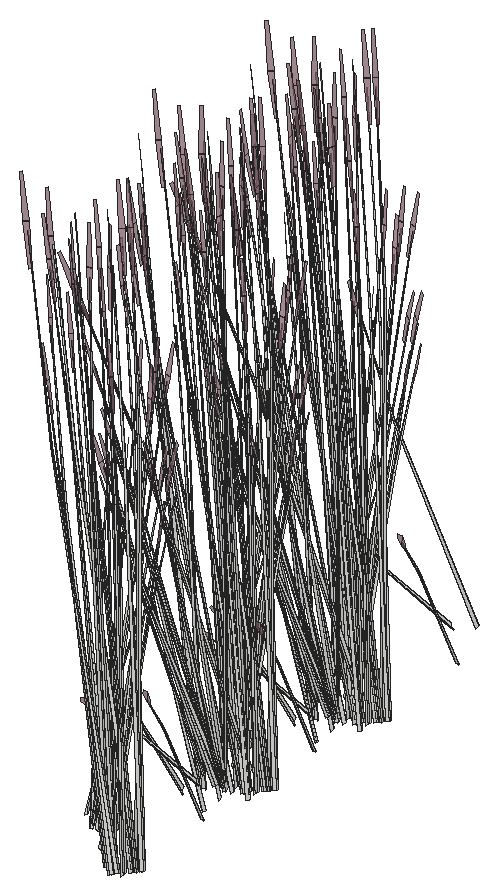
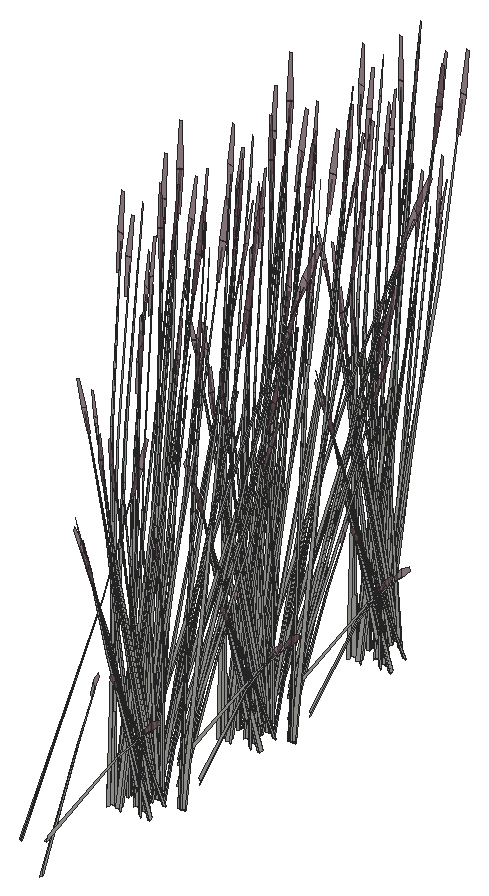
# SketchUp Ruby script. Lengths in inches.
U = 1.inch
M = Sketchup.active_model
def pt(a) = Geom::Point3d.new(a.map { |v| v * U })
def face(e, loops, mat)
  f = e.add_face(loops[0].map { |a| pt(a) })
  loops[1..].each { |l| e.add_face(l.map { |a| pt(a) }).erase! }
  f.material = f.back_material = mat if mat
  f
end
# faces: each face lists its corners as indices into pts; further lists are holes
def faces(e, pts, list, mat = nil) = list.each { |f| face(e, (f[0].is_a?(Array) ? f : [f]).map { |l| l.map { |i| pts[i] } }, mat) }
# xy, xz, yz: faces in a plane at the given z, y or x. An outline is a flat list of corners, or four numbers for a rectangle; further outlines are holes
def ring(l) = l.size == 4 ? [[l[0], l[1]], [l[2], l[1]], [l[2], l[3]], [l[0], l[3]]] : l.each_slice(2).to_a
def flat(e, list, mat, &to3) = list.each { |f| face(e, (f[0].is_a?(Array) ? f : [f]).map { |l| ring(l).map { |u, v| to3.(u, v) } }, mat) }
def xy(e, z, list, mat = nil) = flat(e, list, mat) { |x, y| [x, y, z] }
def xz(e, y, list, mat = nil) = flat(e, list, mat) { |x, z| [x, y, z] }
def yz(e, x, list, mat = nil) = flat(e, list, mat) { |y, z| [x, y, z] }
def lines(e, pts, list) = list.each { |a, b| e.add_line(pt(pts[a]), pt(pts[b])) }
# prism: a flat outline (further loops are holes) pulled along v
def prism(e, loops, v, mat = nil)
  f = face(e, loops, mat); d = Geom::Vector3d.new(v.map { |x| x * U })
  f.pushpull(f.normal.samedirection?(d) ? d.length : -d.length)
end
def box(e, o, s, mat = nil) = prism(e, [[o, [o[0] + s[0], o[1], o[2]], [o[0] + s[0], o[1] + s[1], o[2]], [o[0], o[1] + s[1], o[2]]]], [0, 0, s[2]], mat)
def at(x, y, z, deg = 0) = Geom::Transformation.translation(pt([x, y, z])) * Geom::Transformation.rotation(ORIGIN, Z_AXIS, deg.degrees)
def axes(o, x, y, z) = Geom::Transformation.new([*x, 0, *y, 0, *z, 0, *pt(o).to_a, 1])
def part(name) = M.definitions.add(name)
# library, detail: a bought-in or finely detailed component or shape, given as its bounding box
def library(name, o, s) = part(name).tap { |d| box(d.entities, o, s) }
def detail(e, o, s) = box(e.add_group.entities, o, s)
def put(e, d, t, mat = nil) = e.add_instance(d, t).tap { |i| i.material = mat if mat }
def group(e, t, mat = nil) = e.add_group.tap { |g| g.transformation = t; g.material = mat if mat }.entities
root = M.entities
M.materials.add("LightPink_Translucent").color = [144, 107, 117]
M.materials["LightPink_Translucent"].alpha = 0.75
c1 = part("blade")
p = [[2.15,0.21,22],[0,0.17,0],[0.09,0.45,0],[2.18,0.31,22],[2.29,0.31,22],[0.38,0.45,0],
  [2.48,0.24,33],[2.49,0.24,33],[2.48,0.22,33]]
faces(c1.entities,p,[[0,1,2,3],[4,5,2,3],[6,3,4,7],[8,0,3,6]])
c2 = part("seeds")
p = [[0.3,-0.1,1.38],[-0.01,-0.03,1.59],[-0.01,-0.03,0.03],[0.14,-0.07,-0.07],[0.29,-0.03,3],[0.15,0.01,3.11]]
faces(c2.entities,p,[[0,1,2,3],[1,0,4,5]],"LightPink_Translucent")
c3 = part("blade with seeds")
put(c3.entities,c1,at(0,0,0))
put(c3.entities,c2,axes([2.4,0.25,30.99],[1.5799,-0.05474,1.17369],[-0.12525,1.92788,0.29478],[-0.07173,-0.02425,1.56792]))
put(root,c3,axes([343.19,119.87,4.77],[0.96132,-0.17317,0.17642],[0.23737,0.64447,0.35086],[-0.08574,-0.0939,1.60407]))
put(root,c3,axes([344.08,119.18,4.91],[-0.17258,0.58229,0.1448],[-0.84319,-0.10108,-0.41347],[-0.15345,-0.05979,1.26744]))
put(root,c3,axes([346.05,119.9,4.77],[0.25843,-0.64844,0.17642],[0.9457,0.1835,0.35086],[-0.16336,0.00316,1.60407]))
put(root,c3,axes([344.43,119.97,4.49],[-0.90188,-0.29293,0],[0.43405,-0.60866,0],[0,0,1.62707]))
put(root,c3,axes([345.18,119.19,4.76],[-0.87356,-0.52515,-0.25192],[0.73507,-0.5897,0.5513],[-0.23523,0.06143,1.68216]))
put(root,c3,axes([342.88,120.2,4.77],[0.83726,0.32623,0.49651],[-0.50045,0.58498,0],[-0.19069,-0.0743,1.57504]))
put(root,c3,axes([345.6,118.76,5.01],[0.97146,-0.04028,0.44739],[0.08785,0.66859,-0.21531],[-0.17391,0.06776,1.43643]))
put(root,c3,axes([344.74,119.08,4.5],[-0.97146,0.04028,-0.44739],[-0.08785,-0.66859,0.21531],[-0.17391,0.06776,1.43643]))
put(root,c3,axes([345.8125,120.63,4.49],[-0.55235,-0.65609,-0.05142],[0.93577,-0.36461,0.51607],[-0.23059,0.06247,1.6363]))
put(root,c3,axes([345.62,119.04,4.91],[0.66093,0.39201,0.1448],[-0.5513,0.44227,-0.41347],[-0.15345,0.05979,1.26744]))
put(root,c3,axes([346.32,120.25,4.77],[0.83726,-0.32623,0.49651],[0.50045,0.58498,0],[-0.19069,0.0743,1.57504]))
put(root,c3,axes([345.5625,120.55,4.32],[-0.83462,-0.16144,-0.30978],[0.21015,-0.56852,0.30978],[-0.16826,0.06556,1.38974]))
put(root,c3,axes([345.42,118.9,4.96],[0.10425,0.7445,-0.29095],[-1.08575,0.04502,-0.50002],[-0.19119,0.09917,1.59708]))
put(root,c3,axes([344.77,119.47,4.35],[-0.60257,0.49041,-0.62353],[-0.74854,-0.44469,-0.16365],[-0.24146,0.12234,1.37633]))
put(root,c3,axes([345.84,120.29,4.625],[1.11998,0.21207,0.30756],[-0.2802,0.75803,-0.36492],[-0.18537,0.09487,1.64885]))
put(root,c3,axes([345.76,120.8,4.3125],[-0.83726,0.32623,-0.49651],[-0.50045,-0.58498,0],[-0.19069,0.0743,1.57504]))
put(root,c3,axes([341.98,120.01,7.34],[0.60531,-0.34352,0.35414],[0.573,0.39225,-0.4572],[-0.08718,0.19929,0.87481]))
put(root,c3,axes([346.52,120.7,4.67],[0.55932,0.6538,0],[-0.93577,0.36461,-0.51607],[-0.21313,0.08304,1.63711]))
put(root,c3,axes([346.04,118.12,5.13],[-0.02444,-0.61432,1.41272],[1.10603,0.15924,0.59816],[-0.26159,0.33615,1.3335]))
put(root,c3,axes([343.4375,121.03,7.02],[-0.6592,0.22175,0.0643],[-0.32265,-0.40436,0.50621],[0.06366,0.17825,0.77189]))
put(root,c3,axes([341.67,120.49,6.82],[-0.60531,0.34352,-0.35414],[-0.573,-0.39225,0.4572],[-0.08718,0.19929,0.87481]))
put(root,c3,axes([341.6,120.1,7.69],[0.98321,0.03233,-0.13498],[-0.02687,0.61208,-0.74919],[-0.0683,0.23574,1.13838]))
put(root,c3,axes([343.67,120.98,7.36],[-0.88151,-0.17057,0.53283],[0.30143,-0.56078,0.43934],[0.05297,0.22053,1.10256]))
put(root,c3,axes([342.05,121.83,5.06],[-0.02315,-0.38796,1.1486],[0.57853,0.27671,0.84392],[-0.11378,0.18492,0.25299]))
put(root,c3,axes([342.27,120.33,7.3],[0.64041,0.4384,-0.5672],[-0.67652,0.38394,-0.43934],[-0.09744,0.22274,1.08528]))
put(root,c3,axes([341.57,120.99,5.12],[0.8127,-0.11554,0.06507],[0.18684,0.46549,-0.86304],[-0.05152,0.23564,0.7736]))
put(root,c3,axes([342.07,120.13,7.63],[-0.02328,0.60353,-0.7886],[-0.98022,-0.04053,0.09517],[-0.10344,0.25568,1.11556]))
put(root,c3,axes([339.51,121.72,7],[0.10149,-0.03939,1.77383],[0.83886,0.26202,-0.16761],[-0.01971,0.21816,0.31391]))
put(root,c3,axes([343,119.7,6.17],[-0.0219,-0.25042,1.71376],[0.94901,0.16613,0.13857],[-0.0587,0.35688,0.73262]))
put(root,c3,axes([343.98,131.05,7.01],[-0.13683,-0.09148,1.74944],[-0.91315,0.058,-0.27667],[-0.14574,-0.2188,0.14031]))
put(root,c3,axes([341.74,120.98,5.66],[0.01966,-0.33682,1.54345],[0.88405,0.17791,0.21329],[-0.0766,0.35897,0.72882]))
put(root,c3,axes([344.94,132.59,7.27],[-0.42698,-0.53052,-0.71045],[0.87893,-0.29566,0.08574],[-0.09984,-0.25633,1.00501]))
put(root,c3,axes([344.2,131.42,3.79],[-0.15005,0.02351,1.76342],[-0.82981,-0.26461,-0.26939],[0.01392,-0.22072,0.30037]))
put(root,c3,axes([345.02,132.14,6.82],[0.2697,-0.50175,-0.35414],[0.78684,0.14635,0.4572],[-0.07215,-0.20201,0.87481]))
put(root,c3,axes([344.62,132.49,6.97],[-0.87941,-0.16356,-0.51099],[0.30143,-0.56078,-0.3958],[-0.08064,-0.22578,0.97773]))
put(root,c3,axes([342.87,132.14,7.39],[0.99656,-0.1677,0.53763],[0.17295,0.65785,0.4433],[-0.23438,-0.19388,1.11249]))
put(root,c3,axes([345.37,132.46,7.33],[-0.87543,0.30377,-0.1216],[-0.4302,-0.53915,-0.67495],[-0.1155,-0.2272,1.02557]))
put(root,c3,axes([341.89,131.54,5.06],[0.46666,0.22709,1.1486],[-0.67962,0.13651,0.84392],[-0.14541,-0.17452,0.25299]))
put(root,c3,axes([343.09,132.28,7.02],[0.4066,-0.41448,0.0643],[0.57901,0.24131,0.50621],[-0.18719,-0.13288,0.77189]))
put(root,c3,axes([342.97,134.59,4.39],[-0.36739,-0.66907,-0.69835],[1.05831,-0.24096,-0.18329],[-0.04061,-0.22656,1.54149]))
put(root,c3,axes([345.11,132.67,7.34],[-0.2697,0.50175,0.35414],[-0.78684,-0.14635,-0.4572],[-0.07215,-0.20201,0.87481]))
put(root,c3,axes([344.05,131.875,4.42],[-0.61821,0.37431,-0.03893],[-0.56645,-0.40995,-0.17649],[-0.03988,-0.11616,0.58215]))
put(root,c3,axes([344.84,136.3125,5.62],[0.77308,0.2631,1.51261],[-0.75736,0.56681,0.59816],[-0.33924,-0.33594,1.26806]))
put(root,c3,axes([343.22,132.76,7.34],[0.13817,0.52554,0.35414],[-0.78985,0.13877,-0.4572],[-0.21215,-0.1506,0.87481]))
put(root,c3,axes([340.8,134.49,4.3125],[0,-0.65246,-0.49651],[1.00089,0,0],[0,-0.1486,1.57504]))
put(root,c3,axes([341.23,134.51,4.32],[0.62448,-0.40708,-0.30978],[0.62448,0.40708,0.30978],[0,-0.13112,1.38974]))
put(root,c3,axes([343.42,135.25,4.96],[-1.00749,-0.31132,-0.29095],[0.48511,-0.65709,-0.50002],[-0.03166,-0.16133,1.59708]))
put(root,c3,axes([341.42,134.8,4.625],[-0.83213,0.54855,0.30756],[-0.83263,-0.54278,-0.36492],[-0.02906,-0.15578,1.64885]))
put(root,c3,axes([343.67,135.94,4.73],[0.23711,-0.77313,-0.23429],[1.12425,0.13477,0.51271],[-0.19645,-0.10677,1.5644]))
put(root,c3,axes([341.23,135.1,4.77],[0,0.65246,0.49651],[-1.00089,0,0],[0,-0.1486,1.57504]))
put(root,c3,axes([343.59,135.625,4.5],[-0.53742,-0.54764,-0.44739],[0.81403,-0.38564,0.21531],[-0.17391,-0.06776,1.43643]))
put(root,c3,axes([343.7,134.85,4.65],[0.38895,0.72959,0.45755],[-1.11135,0.2537,0.17955],[0.01358,-0.13406,1.58856]))
put(root,c3,axes([343.51,135.43,5.01],[-0.43405,0.58792,0.44739],[-0.90188,-0.28295,-0.21531],[0,-0.13553,1.43643]))
put(root,c3,axes([345.38,135.5,4.59],[-0.83213,-0.56158,-0.06131],[0.83263,-0.56193,0],[-0.02906,-0.01961,1.75571]))
put(root,c3,axes([343.8,135.57,4.65],[1.13071,0.13747,0.45755],[-0.23011,0.77639,0.17955],[-0.16524,-0.07497,1.58856]))
put(root,c3,axes([343.19,136.81,4.77],[0.96132,-0.17317,0.17642],[0.23737,0.64447,0.35086],[-0.08574,-0.0939,1.60407]))
put(root,c3,axes([344.08,136.12,4.91],[-0.17258,0.58229,0.1448],[-0.84319,-0.10108,-0.41347],[-0.15345,-0.05979,1.26744]))
put(root,c3,axes([346.05,136.84,4.77],[0.25843,-0.64844,0.17642],[0.9457,0.1835,0.35086],[-0.16336,0.00316,1.60407]))
put(root,c3,axes([344.43,136.91,4.49],[-0.90188,-0.29293,0],[0.43405,-0.60866,0],[0,0,1.62707]))
put(root,c3,axes([345.18,136.13,4.76],[-0.87356,-0.52515,-0.25192],[0.73507,-0.5897,0.5513],[-0.23523,0.06143,1.68216]))
put(root,c3,axes([342.88,137.14,4.77],[0.83726,0.32623,0.49651],[-0.50045,0.58498,0],[-0.19069,-0.0743,1.57504]))
put(root,c3,axes([345.6,135.7,5.01],[0.97146,-0.04028,0.44739],[0.08785,0.66859,-0.21531],[-0.17391,0.06776,1.43643]))
put(root,c3,axes([344.74,136.02,4.5],[-0.97146,0.04028,-0.44739],[-0.08785,-0.66859,0.21531],[-0.17391,0.06776,1.43643]))
put(root,c3,axes([345.8125,137.57,4.49],[-0.55235,-0.65609,-0.05142],[0.93577,-0.36461,0.51607],[-0.23059,0.06247,1.6363]))
put(root,c3,axes([345.62,135.98,4.91],[0.66093,0.39201,0.1448],[-0.5513,0.44227,-0.41347],[-0.15345,0.05979,1.26744]))
put(root,c3,axes([346.32,137.19,4.77],[0.83726,-0.32623,0.49651],[0.50045,0.58498,0],[-0.19069,0.0743,1.57504]))
put(root,c3,axes([345.5625,137.49,4.32],[-0.83462,-0.16144,-0.30978],[0.21015,-0.56852,0.30978],[-0.16826,0.06556,1.38974]))
put(root,c3,axes([345.42,135.84,4.96],[0.10425,0.7445,-0.29095],[-1.08575,0.04502,-0.50002],[-0.19119,0.09917,1.59708]))
put(root,c3,axes([344.77,136.41,4.35],[-0.60257,0.49041,-0.62353],[-0.74854,-0.44469,-0.16365],[-0.24146,0.12234,1.37633]))
put(root,c3,axes([345.84,137.23,4.625],[1.11998,0.21207,0.30756],[-0.2802,0.75803,-0.36492],[-0.18537,0.09487,1.64885]))
put(root,c3,axes([345.76,137.74,4.3125],[-0.83726,0.32623,-0.49651],[-0.50045,-0.58498,0],[-0.19069,0.0743,1.57504]))
put(root,c3,axes([341.98,136.95,7.34],[0.60531,-0.34352,0.35414],[0.573,0.39225,-0.4572],[-0.08718,0.19929,0.87481]))
put(root,c3,axes([346.52,137.64,4.67],[0.55932,0.6538,0],[-0.93577,0.36461,-0.51607],[-0.21313,0.08304,1.63711]))
put(root,c3,axes([346.04,135.06,5.13],[-0.02444,-0.61432,1.41272],[1.10603,0.15924,0.59816],[-0.26159,0.33615,1.3335]))
put(root,c3,axes([341.4375,137.26,7.02],[-0.73517,-0.0304,0.0643],[0.02016,-0.45906,0.50621],[-0.07693,0.17585,0.77189]))
put(root,c3,axes([343.98,145.4,7.01],[-0.13683,-0.09148,1.74944],[-0.91315,0.058,-0.27667],[-0.14574,-0.2188,0.14031]))
put(root,c3,axes([343.4375,137.97,7.02],[-0.6592,0.22175,0.0643],[-0.32265,-0.40436,0.50621],[0.06366,0.17825,0.77189]))
put(root,c3,axes([341.67,137.43,6.82],[-0.60531,0.34352,-0.35414],[-0.573,-0.39225,0.4572],[-0.08718,0.19929,0.87481]))
put(root,c3,axes([344.94,146.94,7.27],[-0.42698,-0.53052,-0.71045],[0.87893,-0.29566,0.08574],[-0.09984,-0.25633,1.00501]))
put(root,c3,axes([341.6,137.04,7.69],[0.98321,0.03233,-0.13498],[-0.02687,0.61208,-0.74919],[-0.0683,0.23574,1.13838]))
put(root,c3,axes([343.67,137.92,7.36],[-0.88151,-0.17057,0.53283],[0.30143,-0.56078,0.43934],[0.05297,0.22053,1.10256]))
put(root,c3,axes([342.05,138.77,5.06],[-0.02315,-0.38796,1.1486],[0.57853,0.27671,0.84392],[-0.11378,0.18492,0.25299]))
put(root,c3,axes([344.2,145.76,3.79],[-0.15005,0.02351,1.76342],[-0.82981,-0.26461,-0.26939],[0.01392,-0.22072,0.30037]))
put(root,c3,axes([342.27,137.27,7.3],[0.64041,0.4384,-0.5672],[-0.67652,0.38394,-0.43934],[-0.09744,0.22274,1.08528]))
put(root,c3,axes([341.57,137.93,5.12],[0.8127,-0.11554,0.06507],[0.18684,0.46549,-0.86304],[-0.05152,0.23564,0.7736]))
put(root,c3,axes([345.02,146.49,6.82],[0.2697,-0.50175,-0.35414],[0.78684,0.14635,0.4572],[-0.07215,-0.20201,0.87481]))
put(root,c3,axes([344.62,146.84,6.97],[-0.87941,-0.16356,-0.51099],[0.30143,-0.56078,-0.3958],[-0.08064,-0.22578,0.97773]))
put(root,c3,axes([342.07,137.07,7.63],[-0.02328,0.60353,-0.7886],[-0.98022,-0.04053,0.09517],[-0.10344,0.25568,1.11556]))
put(root,c3,axes([339.51,138.66,7],[0.10149,-0.03939,1.77383],[0.83886,0.26202,-0.16761],[-0.01971,0.21816,0.31391]))
put(root,c3,axes([343,136.64,6.17],[-0.0219,-0.25042,1.71376],[0.94901,0.16613,0.13857],[-0.0587,0.35688,0.73262]))
put(root,c3,axes([342.87,146.48,7.39],[0.99656,-0.1677,0.53763],[0.17295,0.65785,0.4433],[-0.23438,-0.19388,1.11249]))
put(root,c3,axes([345.37,146.81,7.33],[-0.87543,0.30377,-0.1216],[-0.4302,-0.53915,-0.67495],[-0.1155,-0.2272,1.02557]))
put(root,c3,axes([341.89,145.89,5.06],[0.46666,0.22709,1.1486],[-0.67962,0.13651,0.84392],[-0.14541,-0.17452,0.25299]))
put(root,c3,axes([343.09,146.625,7.02],[0.4066,-0.41448,0.0643],[0.57901,0.24131,0.50621],[-0.18719,-0.13288,0.77189]))
put(root,c3,axes([342.97,148.93,4.39],[-0.36739,-0.66907,-0.69835],[1.05831,-0.24096,-0.18329],[-0.04061,-0.22656,1.54149]))
put(root,c3,axes([341.74,137.92,5.66],[0.01966,-0.33682,1.54345],[0.88405,0.17791,0.21329],[-0.0766,0.35897,0.72882]))
put(root,c3,axes([345.11,147.02,7.34],[-0.2697,0.50175,0.35414],[-0.78684,-0.14635,-0.4572],[-0.07215,-0.20201,0.87481]))
put(root,c3,axes([344.05,146.22,4.42],[-0.61821,0.37431,-0.03893],[-0.56645,-0.40995,-0.17649],[-0.03988,-0.11616,0.58215]))
put(root,c3,axes([344.84,150.66,5.62],[0.77308,0.2631,1.51261],[-0.75736,0.56681,0.59816],[-0.33924,-0.33594,1.26806]))
put(root,c3,axes([343.22,147.1,7.34],[0.13817,0.52554,0.35414],[-0.78985,0.13877,-0.4572],[-0.21215,-0.1506,0.87481]))
put(root,c3,axes([340.8,148.84,4.3125],[0,-0.65246,-0.49651],[1.00089,0,0],[0,-0.1486,1.57504]))
put(root,c3,axes([341.23,148.86,4.32],[0.62448,-0.40708,-0.30978],[0.62448,0.40708,0.30978],[0,-0.13112,1.38974]))
put(root,c3,axes([343.42,149.6,4.96],[-1.00749,-0.31132,-0.29095],[0.48511,-0.65709,-0.50002],[-0.03166,-0.16133,1.59708]))
put(root,c3,axes([341.42,149.14,4.625],[-0.83213,0.54855,0.30756],[-0.83263,-0.54278,-0.36492],[-0.02906,-0.15578,1.64885]))
put(root,c3,axes([343.67,150.29,4.73],[0.23711,-0.77313,-0.23429],[1.12425,0.13477,0.51271],[-0.19645,-0.10677,1.5644]))
put(root,c3,axes([341.23,149.45,4.77],[0,0.65246,0.49651],[-1.00089,0,0],[0,-0.1486,1.57504]))
put(root,c3,axes([343.59,149.97,4.5],[-0.53742,-0.54764,-0.44739],[0.81403,-0.38564,0.21531],[-0.17391,-0.06776,1.43643]))
put(root,c3,axes([343.7,149.2,4.65],[0.38895,0.72959,0.45755],[-1.11135,0.2537,0.17955],[0.01358,-0.13406,1.58856]))
put(root,c3,axes([343.51,149.77,5.01],[-0.43405,0.58792,0.44739],[-0.90188,-0.28295,-0.21531],[0,-0.13553,1.43643]))
put(root,c3,axes([345.38,149.85,4.59],[-0.83213,-0.56158,-0.06131],[0.83263,-0.56193,0],[-0.02906,-0.01961,1.75571]))
put(root,c3,axes([343.8,149.91,4.65],[1.13071,0.13747,0.45755],[-0.23011,0.77639,0.17955],[-0.16524,-0.07497,1.58856]))
put(root,c3,axes([343.19,151.16,4.77],[0.96132,-0.17317,0.17642],[0.23737,0.64447,0.35086],[-0.08574,-0.0939,1.60407]))
put(root,c3,axes([344.08,150.47,4.91],[-0.17258,0.58229,0.1448],[-0.84319,-0.10108,-0.41347],[-0.15345,-0.05979,1.26744]))
put(root,c3,axes([346.05,151.19,4.77],[0.25843,-0.64844,0.17642],[0.9457,0.1835,0.35086],[-0.16336,0.00316,1.60407]))
put(root,c3,axes([344.43,151.26,4.49],[-0.90188,-0.29293,0],[0.43405,-0.60866,0],[0,0,1.62707]))
put(root,c3,axes([345.18,150.48,4.76],[-0.87356,-0.52515,-0.25192],[0.73507,-0.5897,0.5513],[-0.23523,0.06143,1.68216]))
put(root,c3,axes([342.88,151.48,4.77],[0.83726,0.32623,0.49651],[-0.50045,0.58498,0],[-0.19069,-0.0743,1.57504]))
put(root,c3,axes([345.6,150.04,5.01],[0.97146,-0.04028,0.44739],[0.08785,0.66859,-0.21531],[-0.17391,0.06776,1.43643]))
put(root,c3,axes([344.74,150.37,4.5],[-0.97146,0.04028,-0.44739],[-0.08785,-0.66859,0.21531],[-0.17391,0.06776,1.43643]))
put(root,c3,axes([345.8125,151.92,4.49],[-0.55235,-0.65609,-0.05142],[0.93577,-0.36461,0.51607],[-0.23059,0.06247,1.6363]))
put(root,c3,axes([345.62,150.33,4.91],[0.66093,0.39201,0.1448],[-0.5513,0.44227,-0.41347],[-0.15345,0.05979,1.26744]))
put(root,c3,axes([346.32,151.54,4.77],[0.83726,-0.32623,0.49651],[0.50045,0.58498,0],[-0.19069,0.0743,1.57504]))
put(root,c3,axes([345.5625,151.83,4.32],[-0.83462,-0.16144,-0.30978],[0.21015,-0.56852,0.30978],[-0.16826,0.06556,1.38974]))
put(root,c3,axes([345.42,150.19,4.96],[0.10425,0.7445,-0.29095],[-1.08575,0.04502,-0.50002],[-0.19119,0.09917,1.59708]))
put(root,c3,axes([344.77,150.75,4.35],[-0.60257,0.49041,-0.62353],[-0.74854,-0.44469,-0.16365],[-0.24146,0.12234,1.37633]))
put(root,c3,axes([345.84,151.58,4.625],[1.11998,0.21207,0.30756],[-0.2802,0.75803,-0.36492],[-0.18537,0.09487,1.64885]))
put(root,c3,axes([345.76,152.09,4.3125],[-0.83726,0.32623,-0.49651],[-0.50045,-0.58498,0],[-0.19069,0.0743,1.57504]))
put(root,c3,axes([341.98,151.3,7.34],[0.60531,-0.34352,0.35414],[0.573,0.39225,-0.4572],[-0.08718,0.19929,0.87481]))
put(root,c3,axes([346.52,151.99,4.67],[0.55932,0.6538,0],[-0.93577,0.36461,-0.51607],[-0.21313,0.08304,1.63711]))
put(root,c3,axes([346.04,149.4,5.13],[-0.02444,-0.61432,1.41272],[1.10603,0.15924,0.59816],[-0.26159,0.33615,1.3335]))
put(root,c3,axes([341.4375,151.61,7.02],[-0.73517,-0.0304,0.0643],[0.02016,-0.45906,0.50621],[-0.07693,0.17585,0.77189]))
put(root,c3,axes([343.4375,152.31,7.02],[-0.6592,0.22175,0.0643],[-0.32265,-0.40436,0.50621],[0.06366,0.17825,0.77189]))
put(root,c3,axes([341.67,151.78,6.82],[-0.60531,0.34352,-0.35414],[-0.573,-0.39225,0.4572],[-0.08718,0.19929,0.87481]))
put(root,c3,axes([341.6,151.39,7.69],[0.98321,0.03233,-0.13498],[-0.02687,0.61208,-0.74919],[-0.0683,0.23574,1.13838]))
put(root,c3,axes([343.67,152.27,7.36],[-0.88151,-0.17057,0.53283],[0.30143,-0.56078,0.43934],[0.05297,0.22053,1.10256]))
put(root,c3,axes([342.05,153.12,5.06],[-0.02315,-0.38796,1.1486],[0.57853,0.27671,0.84392],[-0.11378,0.18492,0.25299]))
put(root,c3,axes([342.27,151.62,7.3],[0.64041,0.4384,-0.5672],[-0.67652,0.38394,-0.43934],[-0.09744,0.22274,1.08528]))
put(root,c3,axes([341.57,152.28,5.12],[0.8127,-0.11554,0.06507],[0.18684,0.46549,-0.86304],[-0.05152,0.23564,0.7736]))
put(root,c3,axes([342.07,151.42,7.63],[-0.02328,0.60353,-0.7886],[-0.98022,-0.04053,0.09517],[-0.10344,0.25568,1.11556]))
put(root,c3,axes([339.51,153,7],[0.10149,-0.03939,1.77383],[0.83886,0.26202,-0.16761],[-0.01971,0.21816,0.31391]))
put(root,c3,axes([343,150.99,6.17],[-0.0219,-0.25042,1.71376],[0.94901,0.16613,0.13857],[-0.0587,0.35688,0.73262]))
put(root,c3,axes([341.74,152.27,5.66],[0.01966,-0.33682,1.54345],[0.88405,0.17791,0.21329],[-0.0766,0.35897,0.72882]))
put(root,c3,axes([343.98,163.5625,7.01],[-0.13683,-0.09148,1.74944],[-0.91315,0.058,-0.27667],[-0.14574,-0.2188,0.14031]))
put(root,c3,axes([344.94,165.11,7.27],[-0.42698,-0.53052,-0.71045],[0.87893,-0.29566,0.08574],[-0.09984,-0.25633,1.00501]))
put(root,c3,axes([344.2,163.93,3.79],[-0.15005,0.02351,1.76342],[-0.82981,-0.26461,-0.26939],[0.01392,-0.22072,0.30037]))
